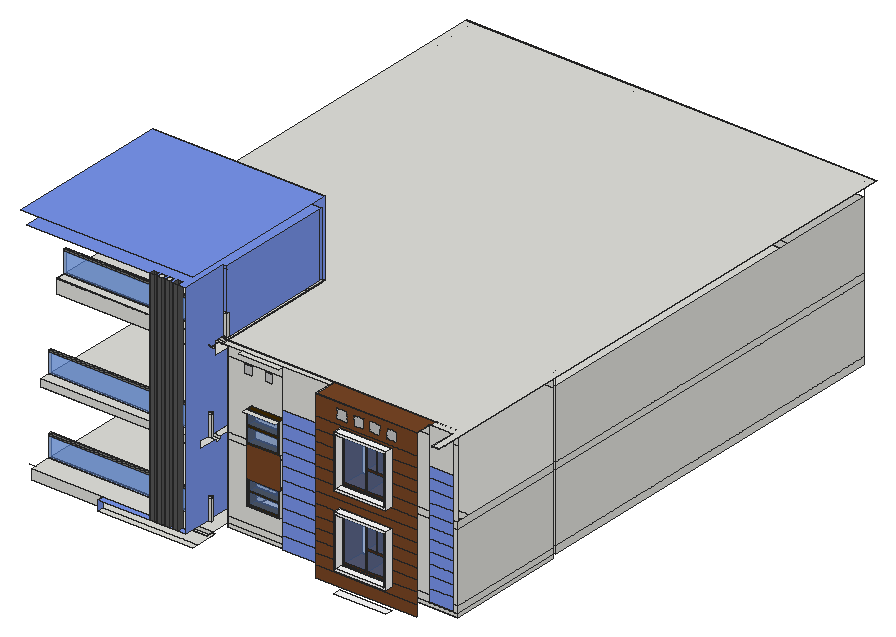
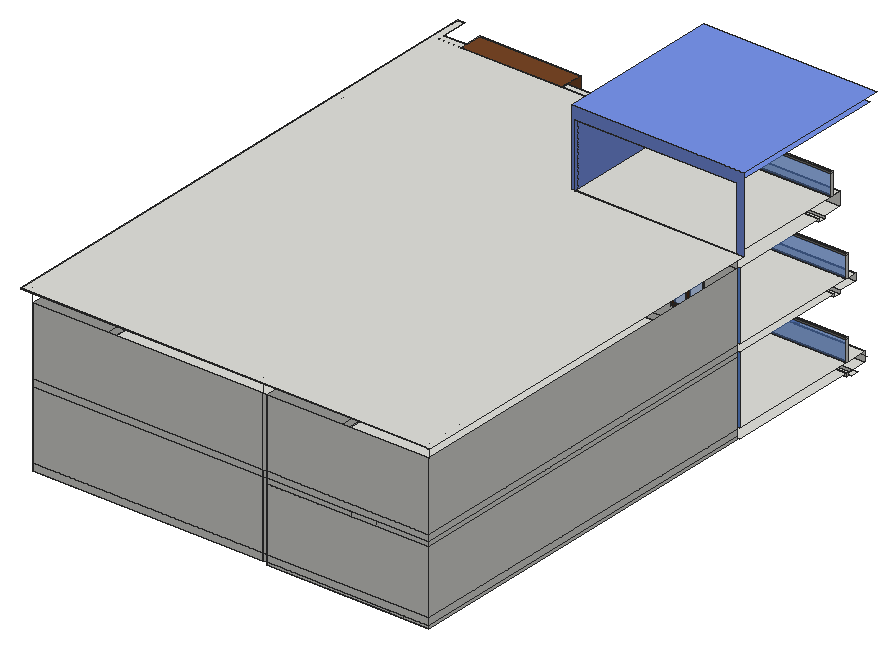
# SketchUp Ruby script. Lengths in inches.
U = 1.inch
M = Sketchup.active_model
def pt(a) = Geom::Point3d.new(a.map { |v| v * U })
def face(e, loops, mat)
  f = e.add_face(loops[0].map { |a| pt(a) })
  loops[1..].each { |l| e.add_face(l.map { |a| pt(a) }).erase! }
  f.material = f.back_material = mat if mat
  f
end
# faces: each face lists its corners as indices into pts; further lists are holes
def faces(e, pts, list, mat = nil) = list.each { |f| face(e, (f[0].is_a?(Array) ? f : [f]).map { |l| l.map { |i| pts[i] } }, mat) }
# xy, xz, yz: faces in a plane at the given z, y or x. An outline is a flat list of corners, or four numbers for a rectangle; further outlines are holes
def ring(l) = l.size == 4 ? [[l[0], l[1]], [l[2], l[1]], [l[2], l[3]], [l[0], l[3]]] : l.each_slice(2).to_a
def flat(e, list, mat, &to3) = list.each { |f| face(e, (f[0].is_a?(Array) ? f : [f]).map { |l| ring(l).map { |u, v| to3.(u, v) } }, mat) }
def xy(e, z, list, mat = nil) = flat(e, list, mat) { |x, y| [x, y, z] }
def xz(e, y, list, mat = nil) = flat(e, list, mat) { |x, z| [x, y, z] }
def yz(e, x, list, mat = nil) = flat(e, list, mat) { |y, z| [x, y, z] }
def lines(e, pts, list) = list.each { |a, b| e.add_line(pt(pts[a]), pt(pts[b])) }
# prism: a flat outline (further loops are holes) pulled along v
def prism(e, loops, v, mat = nil)
  f = face(e, loops, mat); d = Geom::Vector3d.new(v.map { |x| x * U })
  f.pushpull(f.normal.samedirection?(d) ? d.length : -d.length)
end
def box(e, o, s, mat = nil) = prism(e, [[o, [o[0] + s[0], o[1], o[2]], [o[0] + s[0], o[1] + s[1], o[2]], [o[0], o[1] + s[1], o[2]]]], [0, 0, s[2]], mat)
def at(x, y, z, deg = 0) = Geom::Transformation.translation(pt([x, y, z])) * Geom::Transformation.rotation(ORIGIN, Z_AXIS, deg.degrees)
def axes(o, x, y, z) = Geom::Transformation.new([*x, 0, *y, 0, *z, 0, *pt(o).to_a, 1])
def part(name) = M.definitions.add(name)
# library, detail: a bought-in or finely detailed component or shape, given as its bounding box
def library(name, o, s) = part(name).tap { |d| box(d.entities, o, s) }
def detail(e, o, s) = box(e.add_group.entities, o, s)
def put(e, d, t, mat = nil) = e.add_instance(d, t).tap { |i| i.material = mat if mat }
def group(e, t, mat = nil) = e.add_group.tap { |g| g.transformation = t; g.material = mat if mat }.entities
root = M.entities
M.materials.add("[0101_CornflowerBlue]").color = [121, 149, 237]
M.materials.add("[0101_CornflowerBlue]1").color = [100, 149, 237]
M.materials.add("[0117_GhostWhite]").color = [248, 248, 255]
M.materials.add("[Color C08]").color = [80, 48, 26]
M.materials.add("[Color C08]1").color = [63, 41, 0]
M.materials.add("[Color M00]").color = [255, 255, 255]
M.materials.add("[Color M02]").color = [198, 198, 198]
M.materials.add("[Color M06]").color = [86, 86, 86]
M.materials.add("[Metal Seamed]").color = [118, 119, 115]
M.materials.add("[Translucent Glass Blue]").color = [100, 149, 237]
M.materials["[Translucent Glass Blue]"].alpha = 0.5
M.materials.add("[Wood Veneer 01]").color = [120, 70, 37]
c1 = part("Group\#3")
detail(c1.entities,[0,0,0],[48,6.625,84])
c2 = part("Group\#1")
xy(c2.entities,0,[[0,0,32.9375,6]],"[Color C08]")
xy(c2.entities,1.25,[[1.25,0,16.47,6],[17.37,0,31.6875,6]],"[Color C08]")
xy(c2.entities,14.6,[[17.37,0,31.6875,6]],"[Color C08]")
xy(c2.entities,15.72,[[17.37,0,24.18,6],[24.78,0,31.6875,6]],"[Color C08]")
xy(c2.entities,31.6875,[[1.25,0,16.47,6],[17.37,0,24.18,6],[24.78,0,31.6875,6]],"[Color C08]")
xy(c2.entities,32.9375,[[0,0,32.9375,6]],"[Color C08]")
xz(c2.entities,0,[[[0,0,32.9375,32.9375],[1.25,1.25,16.47,31.6875],[17.37,1.25,31.6875,14.6],[24.78,15.72,31.6875,31.6875],[17.37,15.72,24.18,31.6875]]],"[Color C08]")
xz(c2.entities,0,[[1.25,1.25,16.47,31.6875],[17.37,1.25,31.6875,14.6],[17.37,15.72,24.18,31.6875],[24.78,15.72,31.6875,31.6875]],"[Translucent Glass Blue]")
xz(c2.entities,6,[[[0,0,32.9375,32.9375],[1.25,1.25,16.47,31.6875],[17.37,1.25,31.6875,14.6],[24.78,15.72,31.6875,31.6875],[17.37,15.72,24.18,31.6875]]],"[Color C08]")
yz(c2.entities,0,[[0,0,6,32.9375]],"[Color C08]")
yz(c2.entities,1.25,[[0,1.25,6,31.6875]],"[Color C08]")
yz(c2.entities,16.47,[[0,1.25,6,31.6875]],"[Color C08]")
yz(c2.entities,17.37,[[0,1.25,6,14.6],[0,15.72,6,31.6875]],"[Color C08]")
yz(c2.entities,24.18,[[0,15.72,6,31.6875]],"[Color C08]")
yz(c2.entities,24.78,[[0,15.72,6,31.6875]],"[Color C08]")
yz(c2.entities,31.6875,[[0,1.25,6,14.6],[0,15.72,6,31.6875]],"[Color C08]")
yz(c2.entities,32.9375,[[0,0,6,32.9375]],"[Color C08]")
c3 = part("Group\#2")
xy(c3.entities,0,[[0,0,24.1875,6]])
xy(c3.entities,1.18,[[1.18,0,23.01,6]],"[Color C08]1")
xy(c3.entities,14.41,[[1.18,0,23.01,6]],"[Color C08]1")
xy(c3.entities,15.84,[[1.18,0,23.01,6]],"[Color C08]1")
xy(c3.entities,27.63,[[1.18,0,23.01,6]],"[Color C08]1")
xy(c3.entities,28.8125,[[0,0,24.1875,6]],"[Color C08]1")
xz(c3.entities,0,[[[0,0,24.1875,28.8125],[1.18,1.18,23.01,14.41],[1.18,15.84,23.01,27.63]]],"[Color C08]1")
xz(c3.entities,0,[[1.18,1.18,23.01,14.41],[1.18,15.84,23.01,27.63]],"[Translucent Glass Blue]")
xz(c3.entities,6,[[[0,0,24.1875,28.8125],[1.18,1.18,23.01,14.41],[1.18,15.84,23.01,27.63]]],"[Color C08]1")
yz(c3.entities,0,[[0,0,6,28.8125]],"[Color C08]1")
yz(c3.entities,1.18,[[0,1.18,6,14.41],[0,15.84,6,27.63]],"[Color C08]1")
yz(c3.entities,23.01,[[0,1.18,6,14.41],[0,15.84,6,27.63]],"[Color C08]1")
yz(c3.entities,24.1875,[[0,0,6,28.8125]],"[Color C08]1")
xy(root,365.8125,[[12,37.45,297.1875,50.12]])
xy(root,369.09,[[533.125,21.97,624.63,35.47]],"[Color M00]")
xy(root,370,[[303.1875,75.64,708,284.375]])
xy(root,370.8125,[[136.67,0,303.1875,9.875],[12,9.875,12,37.45,297.1875,37.45,297.1875,48.0625,303.1875,48.0625,303.1875,9.875],[2.88,37.45,12,50.12],[12,50.12,297.1875,284.375]])
xy(root,372,[[12,290.375,297.1875,967.0625]])
xy(root,376,[[303.1875,75.64,708,284.375],[12,290.375,297.1875,967.0625],[303.1875,290.375,708,967.0625]])
xy(root,388,[[240.18,0,248.79,9.875],[253.87,0,262.47,9.875],[12,9.875,290.5625,48.0625],[12,48.0625,297.1875,52.0625],[12,52.0625,290.5625,52.0625,290.5625,284.375,239.66,284.375,239.66,290.375,191.66,290.375,191.66,284.375,12,284.375]])
xy(root,388,[[136.67,0,227.24,9.875],[227.24,0,235.85,9.875],[235.85,0,240.18,9.875],[248.79,0,253.87,9.875],[262.47,0,268.12,9.875],
  [268.12,0,276.72,9.875],[276.72,0,290.5625,9.875]],"[0101_CornflowerBlue]")
xy(root,405.53,[[64.85,280.375,135.35,284.375]],"[0117_GhostWhite]")
xy(root,405.85,[[533.125,21.97,624.63,35.47]],"[Color M00]")
xy(root,408.44,[[69.91,280.375,129.66,284.375]],"[0117_GhostWhite]")
xy(root,409.03,[[71.39,284.375,129.26,290.375]])
xy(root,409.41,[[536.9375,21.97,620.9375,35.47]],"[Color M00]")
xy(root,412.1,[[539.1,35.47,618.73,75.64]])
xy(root,423.38,[[346.17,64.22,403.55,75.64]])
xy(root,424,[[12,48.0625,297.1875,52.0625]])
xy(root,427,[[290.5625,48.0625,297.1875,52.0625]])
xy(root,427,[[12,48.0625,290.5625,52.0625]],"[Metal Seamed]")
xy(root,465.77,[[346.17,64.22,403.55,75.64]],"[Wood Veneer 01]")
xy(root,471.3125,[[191.66,284.375,239.66,290.375]])
xy(root,480.9,[[71.39,284.375,129.26,290.375]])
xy(root,481.9,[[69.91,280.375,129.66,284.375]],"[0117_GhostWhite]")
xy(root,487.78,[[64.85,280.375,135.35,284.375]],"[0117_GhostWhite]")
xy(root,491.72,[[539.1,35.47,618.73,75.64]])
xy(root,494.22,[[536.9375,21.97,620.9375,35.47]],"[Color M00]")
xy(root,498.1,[[533.125,21.97,624.63,35.47]],"[Color M00]")
xy(root,500,[[12,290.375,297.1875,967.0625]])
xy(root,503,[[12,65.23,290.5625,77.9]])
xy(root,508,[[12,31.0625,290.5625,65.23],[12,77.9,290.5625,284.375],[12,290.375,297.1875,967.0625],[303.1875,290.375,708,967.0625]])
xy(root,520,[[12,31.0625,290.5625,48.0625],[12,48.0625,297.1875,52.0625],[12,52.0625,290.5625,52.0625,290.5625,284.375,239.66,284.375,239.66,290.375,191.66,290.375,191.66,284.375,12,284.375]])
xy(root,521.63,[[346.17,64.22,403.55,75.64]],"[Wood Veneer 01]")
xy(root,531.78,[[533.125,21.97,624.63,35.47]],"[Color M00]")
xy(root,535.35,[[536.9375,21.97,620.9375,35.47]],"[Color M00]")
xy(root,537.34,[[64.85,280.375,135.35,284.375]],"[0117_GhostWhite]")
xy(root,538.22,[[539.1,35.47,618.73,75.64]])
xy(root,541.07,[[70.78,280.375,129.97,284.375]],"[0117_GhostWhite]")
xy(root,541.71,[[71.39,284.375,129.26,290.375]])
xy(root,556,[[12,48.0625,297.1875,52.0625]])
xy(root,559,[[290.5625,48.0625,297.1875,52.0625]])
xy(root,559,[[12,48.0625,290.5625,52.0625]],"[Metal Seamed]")
xy(root,575.64,[[346.17,55.09,403.55,64.22],[346.17,64.22,403.55,75.64]])
xy(root,603.3125,[[191.66,284.375,239.66,290.375]])
xy(root,613.59,[[71.39,284.375,129.26,290.375]])
xy(root,613.84,[[70.78,280.375,129.97,284.375]],"[0117_GhostWhite]")
xy(root,617.85,[[539.1,35.47,618.73,75.64]])
xy(root,619.59,[[64.85,280.375,135.35,284.375]],"[0117_GhostWhite]")
xy(root,620.16,[[536.9375,21.97,620.9375,35.47]],"[Color M00]")
xy(root,624.03,[[533.125,21.97,624.63,35.47]],"[Color M00]")
xy(root,635,[[12,97.73,290.5625,110.4]])
xy(root,640,[[12,64.22,290.5625,97.73],[12,110.4,290.5625,284.375]])
xy(root,663.5625,[[12,64.22,290.5625,81.22],[12,81.22,297.1875,85.22],[12,85.22,297.1875,290.375]])
xy(root,664,[[708,19.0625,720,19.0625,720,979.0625,0,979.0625,0,290.375,303.1875,290.375,303.1875,75.64,668.47,75.64,668.47,64.22,708,64.22],[338.82,55.09,410.48,64.22],[303.1875,64.22,491.29,75.64]])
xy(root,664,[[491.29,35.47,668.47,75.64]],"[Wood Veneer 01]")
xy(root,700,[[12,81.22,289.625,85.22],[289.625,81.22,297.1875,85.22]])
xy(root,703,[[12,81.22,297.1875,85.22]],"[Metal Seamed]")
xy(root,775.58,[[240.18,0,248.79,9.875],[253.87,0,262.47,9.875]])
xy(root,775.58,[[12,0,12,290.375,297.1875,290.375,297.1875,81.22,290.5625,81.22,290.5625,0,276.72,0,276.72,9.875,268.12,9.875,268.12,0,262.47,0,262.47,9.875,253.87,9.875,253.87,0,248.79,0,248.79,9.875,240.18,9.875,240.18,0,235.85,0,235.85,9.875,227.24,9.875,227.24,0]],"[0101_CornflowerBlue]")
xy(root,796.1875,[[0,0,303.1875,290.375]],"[0101_CornflowerBlue]")
xz(root,0,[[227.24,388,235.85,775.58],[240.18,388,248.79,775.58],[253.87,388,262.47,775.58],[268.12,388,276.72,775.58]],"[Color M06]")
xz(root,9.875,[[12,370.8125,136.67,388]])
xz(root,9.875,[[227.24,388,235.85,775.58],[240.18,388,248.79,775.58],[253.87,388,262.47,775.58],[268.12,388,276.72,775.58]],"[Color M06]")
xz(root,19.0625,[[708,663.5625,720,664]])
xz(root,21.97,[[[533.125,405.85,624.63,498.1],[536.9375,409.41,620.9375,494.22]],[[533.125,531.78,624.63,624.03],[536.9375,535.35,620.9375,620.16]]],"[Color M00]")
xz(root,31.0625,[[12,508,290.5625,520]])
xz(root,35.47,[[[533.125,531.78,624.63,624.03],[536.9375,535.35,620.9375,620.16]]],"[Color M00]")
xz(root,35.47,[[526.8,635.84,544.49,653.53],[556.55,635.84,574.24,653.53],[584.8,635.84,602.49,653.53],[615.36,635.84,633.05,653.53]],"[Color M02]")
xz(root,35.47,[[491.29,374.34,668.47,393.84],[491.29,393.84,668.47,393.84,668.47,413.34,624.63,413.34,624.63,405.85,533.125,405.85,533.125,413.34,491.29,413.34],[[533.125,405.85,624.63,498.1],[536.9375,409.41,620.9375,494.22]],[536.9375,409.41,620.9375,409.41,620.9375,413.34,618.73,413.34,618.73,412.1,539.1,412.1,539.1,413.34,536.9375,413.34],[491.29,413.34,533.125,432.84],
  [536.9375,413.34,539.1,432.84],[618.73,413.34,620.9375,432.84],[624.63,413.34,668.47,432.84],[491.29,432.84,533.125,452.34],[536.9375,432.84,539.1,452.34],
  [618.73,432.84,620.9375,452.34],[624.63,432.84,668.47,452.34],[491.29,452.34,533.125,471.84],[536.9375,452.34,539.1,471.84],[618.73,452.34,620.9375,471.84],
  [624.63,452.34,668.47,471.84],[491.29,471.84,533.125,491.34],[536.9375,471.84,539.1,491.34],[618.73,471.84,620.9375,491.34],[624.63,471.84,668.47,491.34],
  [491.29,491.34,533.125,491.34,533.125,498.1,624.63,498.1,624.63,491.34,668.47,491.34,668.47,510.84,491.29,510.84],[536.9375,491.34,539.1,491.34,539.1,491.72,618.73,491.72,618.73,491.34,620.9375,491.34,620.9375,494.22,536.9375,494.22],[491.29,510.84,668.47,530.34],[491.29,530.34,668.47,530.34,668.47,549.84,624.63,549.84,624.63,531.78,533.125,531.78,533.125,549.84,491.29,549.84],[536.9375,535.35,620.9375,535.35,620.9375,549.84,618.73,549.84,618.73,538.22,539.1,538.22,539.1,549.84,536.9375,549.84],
  [491.29,549.84,533.125,569.34],[536.9375,549.84,539.1,569.34],[618.73,549.84,620.9375,569.34],[624.63,549.84,668.47,569.34],[491.29,569.34,533.125,588.84],
  [536.9375,569.34,539.1,588.84],[618.73,569.34,620.9375,588.84],[624.63,569.34,668.47,588.84],[491.29,588.84,533.125,608.34],[536.9375,588.84,539.1,608.34],
  [618.73,588.84,620.9375,608.34],[624.63,588.84,668.47,608.34],[491.29,608.34,533.125,608.34,533.125,624.03,624.63,624.03,624.63,608.34,668.47,608.34,668.47,627.84,491.29,627.84],[536.9375,608.34,539.1,608.34,539.1,617.85,618.73,617.85,618.73,608.34,620.9375,608.34,620.9375,620.16,536.9375,620.16],[[491.29,627.84,668.47,663.5625],[526.8,635.84,544.49,653.53],[556.55,635.84,574.24,653.53],[584.8,635.84,602.49,653.53],[615.36,635.84,633.05,653.53]],
  [491.29,663.5625,668.47,664]],"[Wood Veneer 01]")
xz(root,37.45,[[12,365.8125,297.1875,370.8125]])
xz(root,48.0625,[[290.5625,388,297.1875,424],[290.5625,424,297.1875,427],[290.5625,520,297.1875,556],[290.5625,556,297.1875,559],[290.5625,663.5,297.1875,663.5625],
  [297.1875,663.5,303.1875,663.5625]])
xz(root,48.0625,[[12,424,290.5625,427],[12,556,290.5625,559]],"[Metal Seamed]")
xz(root,48.0625,[[12,388,290.5625,424],[12,520,290.5625,556]],"[Translucent Glass Blue]")
xz(root,50.12,[[12,365.8125,297.1875,370.8125]])
xz(root,52.0625,[[290.5625,388,297.1875,424],[290.5625,424,297.1875,427],[290.5625,520,297.1875,556],[290.5625,556,297.1875,559]])
xz(root,52.0625,[[12,424,290.5625,427],[12,556,290.5625,559]],"[Metal Seamed]")
xz(root,52.0625,[[12,388,290.5625,424],[12,520,290.5625,556]],"[Translucent Glass Blue]")
xz(root,55.09,[[350.89,638.14,362.45,651.96],[386.39,638.14,397.95,651.96]],"[Color M02]")
xz(root,64.22,[[410.48,597.65,491.29,664],[668.47,599.91,708,663.5625],[12,640,290.5625,663.5625],[12,663.5625,290.5625,664],[290.5625,663.5625,297.1875,664],
  [668.47,663.5625,708,664]])
xz(root,64.22,[[410.48,376.4,491.29,398.52],[668.47,384.85,708,406.79],[410.48,398.52,491.29,420.65],[668.47,406.79,708,426.1],[410.48,420.65,491.29,442.77],
  [668.47,426.1,708,445.41],[410.48,442.77,491.29,464.9],[668.47,445.41,708,464.72],[668.47,464.72,708,484.04],[410.48,464.9,491.29,487.02],
  [668.47,484.04,708,503.35],[410.48,487.02,491.29,509.15],[668.47,503.35,708,522.66],[410.48,509.15,491.29,531.27],[668.47,522.66,708,541.97],
  [410.48,531.27,491.29,553.4],[668.47,541.97,708,561.29],[410.48,553.4,491.29,575.52],[668.47,561.29,708,580.6],[410.48,575.52,491.29,597.65],
  [668.47,580.6,708,599.91]],"[0101_CornflowerBlue]")
xz(root,64.22,[[346.17,465.77,403.55,521.63]],"[Wood Veneer 01]")
xz(root,65.23,[[12,503,290.5625,508]])
xz(root,75.64,[[303.1875,370,491.29,376],[491.29,370,708,376],[303.1875,376,491.29,388],[491.29,376,708,388],[[303.1875,388,491.29,508],[346.17,423.38,403.55,465.77]],
  [[491.29,388,708,508],[539.1,412.1,618.73,491.72]],[303.1875,508,491.29,520],[491.29,508,708,520],[[303.1875,520,491.29,640],[346.17,521.63,403.55,575.64]],[[491.29,520,708,640],[539.1,538.22,618.73,617.85]],
  [303.1875,640,491.29,658],[491.29,640,708,658],[303.1875,658,491.29,664],[491.29,658,668.47,663.5625],[668.47,658,708,663.5625],
  [491.29,663.5625,668.47,664],[668.47,663.5625,708,664]])
xz(root,77.9,[[12,503,290.5625,508]])
xz(root,81.22,[[290.5625,663.5625,297.1875,664],[290.5625,664,297.1875,700],[290.5625,700,297.1875,703]])
xz(root,81.22,[[290.5625,703,297.1875,775.58]],"[0101_CornflowerBlue]")
xz(root,81.22,[[12,700,290.5625,703]],"[Metal Seamed]")
xz(root,81.22,[[12,664,290.5625,700]],"[Translucent Glass Blue]")
xz(root,85.22,[[12,700,297.1875,703]],"[Metal Seamed]")
xz(root,85.22,[[12,663.5625,297.1875,700]],"[Translucent Glass Blue]")
xz(root,97.73,[[12,635,290.5625,640]])
xz(root,110.4,[[12,635,290.5625,640]])
xz(root,280.375,[[[64.85,405.53,135.35,487.78],[69.91,408.44,129.66,481.9]],[[64.85,537.34,135.35,619.59],[70.78,541.07,129.97,613.84]]],"[0117_GhostWhite]")
xz(root,284.375,[[303.1875,370,708,376],[303.1875,376,708,388],[303.1875,388,708,640],[303.1875,640,708,658]])
xz(root,284.375,[[[12,388,191.66,388,191.66,471.3125,239.66,471.3125,239.66,388,290.5625,388,290.5625,508,12,508],[64.85,405.53,135.35,487.78]],[[12,520,191.66,520,191.66,603.3125,239.66,603.3125,239.66,520,290.5625,520,290.5625,640,12,640],[64.85,537.34,135.35,619.59]],[[70.78,541.07,129.97,613.84],[71.39,541.71,129.26,613.59]]],"[0101_CornflowerBlue]1")
xz(root,290.375,[[12,372,297.1875,376],[12,376,297.1875,388],[303.1875,376,708,388],[303.1875,388,708,508],[12,500,297.1875,508],
  [12,508,297.1875,520],[303.1875,508,708,520],[[12,520,12,640,297.1875,640,297.1875,520,239.66,520,239.66,603.3125,191.66,603.3125,191.66,520],[71.39,541.71,129.26,613.59]],[303.1875,520,708,640],[12,640,297.1875,663.5625],
  [12,663.5625,297.1875,664]])
xz(root,290.375,[[0,664,0,796.1875,303.1875,796.1875,303.1875,664,297.1875,664,297.1875,775.58,12,775.58,12,664]],"[0101_CornflowerBlue]")
xz(root,290.375,[[[12,388,12,500,297.1875,500,297.1875,388,239.66,388,239.66,471.3125,191.66,471.3125,191.66,388],[71.39,409.03,129.26,480.9]]],"[0101_CornflowerBlue]1")
xz(root,967.0625,[[12,372,56.125,376],[56.125,372,81.15,376],[81.15,372,297.1875,376],[12,376,297.1875,388],[297.1875,376,303.1875,388],
  [303.1875,376,708,388],[12,388,297.1875,500],[297.1875,388,303.1875,508],[303.1875,388,708,508],[12,500,105.02,508],
  [105.02,500,146.96,508],[146.96,500,297.1875,508],[12,508,297.1875,520],[297.1875,508,303.1875,520],[303.1875,508,708,520],
  [12,520,297.1875,640],[297.1875,520,303.1875,640],[303.1875,520,708,640]])
xz(root,979.0625,[[0,663.5625,720,664]])
yz(root,12,[[37.45,365.8125,50.12,370.8125],[290.375,372,967.0625,376],[290.375,376,967.0625,388],[48.0625,388,52.0625,424],[290.375,388,967.0625,500],
  [48.0625,424,52.0625,427],[290.375,500,967.0625,508],[290.375,508,967.0625,520],[48.0625,520,52.0625,556],[290.375,520,967.0625,640],
  [48.0625,556,52.0625,559],[64.22,663.5625,81.22,664],[81.22,663.5625,85.22,700],[81.22,700,85.22,703]])
yz(root,64.85,[[280.375,405.53,284.375,487.78],[280.375,537.34,284.375,619.59]],"[0117_GhostWhite]")
yz(root,69.91,[[280.375,408.44,284.375,481.9]],"[0117_GhostWhite]")
yz(root,70.78,[[280.375,541.07,284.375,613.84]],"[0117_GhostWhite]")
yz(root,71.39,[[284.375,409.03,290.375,480.9],[284.375,541.71,290.375,613.59]])
yz(root,129.26,[[284.375,409.03,290.375,480.9],[284.375,541.71,290.375,613.59]])
yz(root,129.66,[[280.375,408.44,284.375,481.9]],"[0117_GhostWhite]")
yz(root,129.97,[[280.375,541.07,284.375,613.84]],"[0117_GhostWhite]")
yz(root,135.35,[[280.375,405.53,284.375,487.78],[280.375,537.34,284.375,619.59]],"[0117_GhostWhite]")
yz(root,136.67,[[0,370.8125,9.875,388]],"[0101_CornflowerBlue]")
yz(root,191.66,[[284.375,388,290.375,471.3125],[284.375,520,290.375,603.3125]])
yz(root,227.24,[[0,388,9.875,775.58]],"[Color M06]")
yz(root,235.85,[[0,388,9.875,775.58]],"[Color M06]")
yz(root,239.66,[[284.375,388,290.375,471.3125],[284.375,520,290.375,603.3125]])
yz(root,240.18,[[0,388,9.875,775.58]],"[Color M06]")
yz(root,248.79,[[0,388,9.875,775.58]],"[Color M06]")
yz(root,253.87,[[0,388,9.875,775.58]],"[Color M06]")
yz(root,262.47,[[0,388,9.875,775.58]],"[Color M06]")
yz(root,268.12,[[0,388,9.875,775.58]],"[Color M06]")
yz(root,276.72,[[0,388,9.875,775.58]],"[Color M06]")
yz(root,290.5625,[[0,388,0,775.58,81.22,775.58,81.22,663.5625,64.22,663.5625,64.22,640,97.73,640,97.73,635,110.4,635,110.4,640,284.375,640,284.375,520,52.0625,520,52.0625,559,48.0625,559,48.0625,520,31.0625,520,31.0625,508,65.23,508,65.23,503,77.9,503,77.9,508,284.375,508,284.375,388,52.0625,388,52.0625,427,48.0625,427,48.0625,388]],"[0101_CornflowerBlue]")
yz(root,297.1875,[[37.45,365.8125,48.0625,370.8125],[48.0625,365.8125,50.12,370.8125],[290.375,372,967.0625,376],[290.375,376,967.0625,388],[48.0625,388,52.0625,424],
  [290.375,388,967.0625,500],[48.0625,424,52.0625,427],[290.375,500,967.0625,508],[290.375,508,967.0625,520],[48.0625,520,52.0625,556],
  [290.375,520,967.0625,640],[48.0625,556,52.0625,559],[48.0625,663.5625,64.22,664],[85.22,663.5625,85.22,700,81.22,700,81.22,664]])
yz(root,297.1875,[[81.22,663.5625,81.22,664,85.22,663.5625],[85.22,663.5625,85.22,703,81.22,703,81.22,775.58,284.32,775.58,284.32,663.5625],[284.32,663.5625,290.375,775.58]],"[0101_CornflowerBlue]")
yz(root,303.1875,[[75.64,370,284.375,376],[75.64,376,284.375,388],[290.375,376,967.0625,388],[75.64,388,284.375,508],[290.375,388,967.0625,508],
  [75.64,508,284.375,520],[290.375,508,967.0625,520],[75.64,520,284.375,640],[75.64,640,284.375,658],[75.64,658,81.22,664],
  [81.22,658,284.375,664],[64.22,663.5625,75.64,664],[284.375,663.5625,290.375,664,284.375,664]])
yz(root,346.17,[[64.22,423.38,75.64,465.77],[64.22,521.63,75.64,575.64]])
yz(root,403.55,[[64.22,423.38,75.64,465.77],[64.22,521.63,75.64,575.64]])
yz(root,491.29,[[64.22,376,75.64,388],[64.22,388,75.64,508],[64.22,508,75.64,520],[64.22,520,75.64,640],[64.22,640,75.64,663.5625],
  [35.47,663.5625,64.22,664],[64.22,663.5625,75.64,664]])
yz(root,533.125,[[21.97,405.85,35.47,498.1],[21.97,531.78,35.47,624.03]],"[Color M00]")
yz(root,536.9375,[[21.97,409.41,35.47,494.22],[21.97,535.35,35.47,620.16]],"[Color M00]")
yz(root,539.1,[[35.47,412.1,75.64,491.72],[35.47,538.22,75.64,617.85]])
yz(root,618.73,[[35.47,412.1,75.64,491.72],[35.47,538.22,75.64,617.85]])
yz(root,620.9375,[[21.97,409.41,35.47,494.22],[21.97,535.35,35.47,620.16]],"[Color M00]")
yz(root,624.63,[[21.97,405.85,35.47,498.1],[21.97,531.78,35.47,624.03]],"[Color M00]")
yz(root,668.47,[[35.47,663.5625,64.22,664]])
yz(root,708,[[75.64,370,284.375,376],[75.64,376,284.375,388],[290.375,376,967.0625,388],[75.64,388,284.375,508],[290.375,388,967.0625,508],
  [75.64,508,284.375,520],[290.375,508,967.0625,520],[290.375,520,967.0625,640],[19.0625,663.5625,64.22,664]])
yz(root,720,[[19.0625,663.5625,31.0625,664],[31.0625,663.5625,979.0625,664]])
p = [[289.625,81.22,664],[289.625,85.22,663.5625],[297.1875,85.22,663.5625],[297.1875,81.22,664],[290.5625,81.22,664],[708,290.375,640],
  [708,290.375,664],[708,967.0625,640],[708,967.0625,664],[303.1875,290.375,640],[303.1875,290.375,664],[303.1875,967.0625,640],
  [303.1875,967.0625,664],[12,967.0625,640],[12,967.0625,664],[303.1875,85.22,663.5625],[12,899.73,664],[12,899.73,663.5625],
  [12,931.6,664],[12,931.6,663.5625],[0,290.375,664],[-0.1875,290.375,664],[303.1875,81.22,664],[303.1875,75.64,663.5625],
  [297.1875,75.64,663.5625],[297.1875,75.64,775.58],[303.1875,75.64,775.58],[303.1875,284.375,663.5625],[12,19.0625,388],[0,19.0625,388],
  [708,284.375,664],[708,284.375,658]]
faces(root,p,[[0,1,2,3,4]])
lines(root,p,[[5,6],[7,8],[9,10],[11,12],[13,14],[15,2],[16,17],[18,19],[20,21],[22,3],[23,24],[25,26],
  [27,15],[28,29],[30,31]])
put(root,c1,axes([191.4,284.375,388],[1.00545,0,0],[0,0.4897,0],[0,0,1]))
put(root,c2,axes([70.47,284.375,409.03],[1.78505,0,0],[0,0.8931,0],[0,0,2.19699]))
put(root,c2,axes([539.1,35.47,412.1],[2.41746,0,0],[0,6.0075,0],[0,0,2.41746]))
put(root,c3,axes([346.22,66.8125,423.38],[2.37,0,0],[0,2.44902,0],[0,0,1.47136]))
put(root,c1,axes([191.4,284.375,520],[1.00545,0,0],[0,0.4897,0],[0,0,1]))
put(root,c3,axes([346.22,64.22,521.63],[2.37,0,0],[0,2.44902,0],[0,0,1.87458]))
put(root,c2,axes([539.1,35.47,538.22],[2.41746,0,0],[0,6.0075,0],[0,0,2.41746]))
put(root,c2,axes([71.39,285.07,542.4],[1.75712,0,0],[0,0.77699,0],[0,0,2.16129]))
